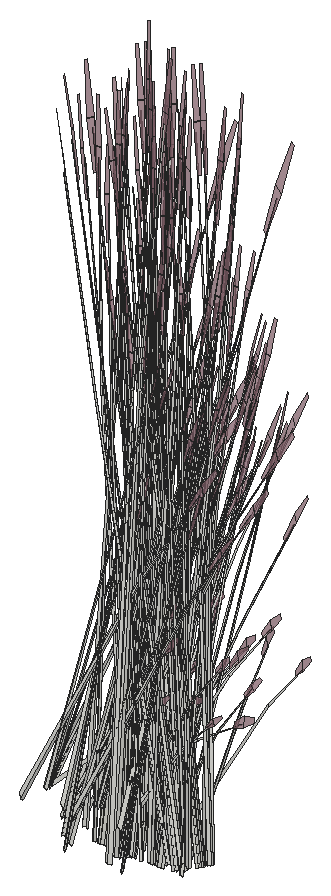
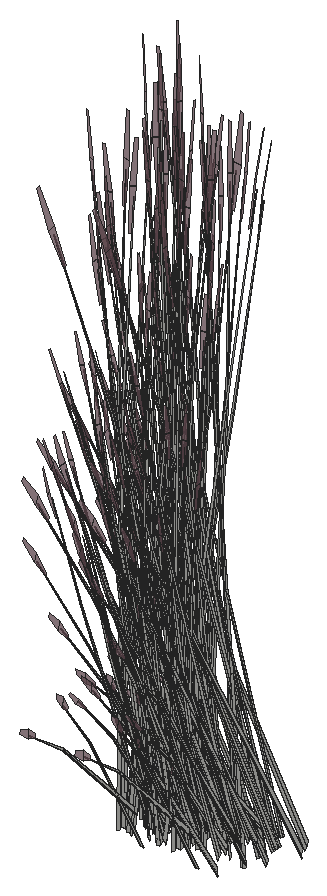
# SketchUp Ruby script. Lengths in inches.
U = 1.inch
M = Sketchup.active_model
def pt(a) = Geom::Point3d.new(a.map { |v| v * U })
def face(e, loops, mat)
  f = e.add_face(loops[0].map { |a| pt(a) })
  loops[1..].each { |l| e.add_face(l.map { |a| pt(a) }).erase! }
  f.material = f.back_material = mat if mat
  f
end
# faces: each face lists its corners as indices into pts; further lists are holes
def faces(e, pts, list, mat = nil) = list.each { |f| face(e, (f[0].is_a?(Array) ? f : [f]).map { |l| l.map { |i| pts[i] } }, mat) }
# xy, xz, yz: faces in a plane at the given z, y or x. An outline is a flat list of corners, or four numbers for a rectangle; further outlines are holes
def ring(l) = l.size == 4 ? [[l[0], l[1]], [l[2], l[1]], [l[2], l[3]], [l[0], l[3]]] : l.each_slice(2).to_a
def flat(e, list, mat, &to3) = list.each { |f| face(e, (f[0].is_a?(Array) ? f : [f]).map { |l| ring(l).map { |u, v| to3.(u, v) } }, mat) }
def xy(e, z, list, mat = nil) = flat(e, list, mat) { |x, y| [x, y, z] }
def xz(e, y, list, mat = nil) = flat(e, list, mat) { |x, z| [x, y, z] }
def yz(e, x, list, mat = nil) = flat(e, list, mat) { |y, z| [x, y, z] }
def lines(e, pts, list) = list.each { |a, b| e.add_line(pt(pts[a]), pt(pts[b])) }
# prism: a flat outline (further loops are holes) pulled along v
def prism(e, loops, v, mat = nil)
  f = face(e, loops, mat); d = Geom::Vector3d.new(v.map { |x| x * U })
  f.pushpull(f.normal.samedirection?(d) ? d.length : -d.length)
end
def box(e, o, s, mat = nil) = prism(e, [[o, [o[0] + s[0], o[1], o[2]], [o[0] + s[0], o[1] + s[1], o[2]], [o[0], o[1] + s[1], o[2]]]], [0, 0, s[2]], mat)
def at(x, y, z, deg = 0) = Geom::Transformation.translation(pt([x, y, z])) * Geom::Transformation.rotation(ORIGIN, Z_AXIS, deg.degrees)
def axes(o, x, y, z) = Geom::Transformation.new([*x, 0, *y, 0, *z, 0, *pt(o).to_a, 1])
def part(name) = M.definitions.add(name)
# library, detail: a bought-in or finely detailed component or shape, given as its bounding box
def library(name, o, s) = part(name).tap { |d| box(d.entities, o, s) }
def detail(e, o, s) = box(e.add_group.entities, o, s)
def put(e, d, t, mat = nil) = e.add_instance(d, t).tap { |i| i.material = mat if mat }
def group(e, t, mat = nil) = e.add_group.tap { |g| g.transformation = t; g.material = mat if mat }.entities
root = M.entities
M.materials.add("LightPink_Translucent").color = [144, 107, 117]
M.materials["LightPink_Translucent"].alpha = 0.75
c1 = part("blade")
p = [[2.15,0.21,22],[0,0.17,0],[0.09,0.45,0],[2.18,0.31,22],[2.29,0.31,22],[0.38,0.45,0],
  [2.48,0.24,33],[2.49,0.24,33],[2.48,0.22,33]]
faces(c1.entities,p,[[0,1,2,3],[4,5,2,3],[6,3,4,7],[8,0,3,6]])
c2 = part("seeds")
p = [[0.3,-0.1,1.38],[-0.01,-0.03,1.59],[-0.01,-0.03,0.03],[0.14,-0.07,-0.07],[0.29,-0.03,3],[0.15,0.01,3.11]]
faces(c2.entities,p,[[0,1,2,3],[1,0,4,5]],"LightPink_Translucent")
c3 = part("blade with seeds")
put(c3.entities,c1,at(0,0,0))
put(c3.entities,c2,axes([2.4,0.25,30.99],[1.5799,-0.05474,1.17369],[-0.12525,1.92788,0.29478],[-0.07173,-0.02425,1.56792]))
put(root,c3,axes([674.73,341.44,393.22],[-0.01592,-0.21915,1.42242],[0.69015,0.14538,0.11501],[-0.04269,0.3123,0.60807]))
put(root,c3,axes([677.3,341.1,393.89],[0.16713,0.52135,-0.42412],[-0.63294,0.0912,-0.32852],[-0.18138,0.14003,0.81151]))
put(root,c3,axes([676.31,342.04,393.91],[-0.01617,0.11299,1.45204],[0.45894,0.39307,-0.22964],[-0.12015,0.18588,0.11645]))
put(root,c3,axes([669.01,340.77,393.22],[-0.24166,-0.09837,1.42242],[0.50011,-0.41269,0.11501],[0.3117,0.18617,0.60807]))
put(root,c3,axes([674.26,340.18,392.06],[0,-0.57097,0.4121],[0.72788,0,0],[0,0.13004,1.30728]))
put(root,c3,axes([674.57,340.71,391.67],[0,0.57097,-0.4121],[-0.72788,0,0],[0,0.13004,1.30728]))
put(root,c3,axes([672.63,342.4375,393.93],[-0.64708,0.13103,0.39842],[-0.1123,-0.514,0.32852],[0.15218,0.15149,0.82444]))
put(root,c3,axes([672.51,342.54,393.93],[-0.29569,0.36271,0.05337],[-0.42107,-0.21117,0.42015],[0.13613,0.11629,0.64067]))
put(root,c3,axes([671.76,341.34,393.22],[-0.14872,-0.18332,1.42242],[0.6872,-0.15433,0.11501],[0.15531,0.28779,0.60807]))
put(root,c3,axes([670.91,340.64,393.93],[0.23895,0.38931,0.05337],[-0.43573,0.19055,0.42015],[0.19208,-0.0376,0.64067]))
put(root,c3,axes([670.33,341.6875,393.76],[0.37017,0.35748,-0.29394],[-0.42268,0.3384,0.37948],[0.21476,0.05149,0.72609]))
put(root,c3,axes([669.91,341.73,394.18],[0.03484,-0.58066,-0.10093],[0.65957,0.01587,-0.56021],[0.25402,0.04034,0.85122]))
put(root,c3,axes([677,340.73,394.18],[0.60181,0.31483,-0.10093],[-0.34671,0.45593,-0.56021],[-0.17003,0.15849,0.85122]))
put(root,c3,axes([670.86,340.51,393.93],[-0.18381,0.5206,0.39842],[-0.60429,-0.17802,0.32852],[0.23764,-0.03129,0.82444]))
put(root,c3,axes([678.36,342.17,391.97],[-0.40676,0.57214,0],[-0.68052,-0.31907,-0.42834],[-0.15499,-0.07267,1.3588]))
put(root,c3,axes([675.77,341.67,391.82],[-0.65588,-0.25634,0],[0.31565,-0.53263,0],[0,0,1.35047]))
put(root,c3,axes([677.29,342.31,391.97],[0.40676,0.57214,0],[-0.68052,0.31907,-0.42834],[-0.15499,0.07267,1.3588]))
put(root,c3,axes([672.53,341.375,391.8125],[0.68303,-0.19373,-0.15934],[0.24001,0.55805,0.00007],[0.07539,-0.02141,1.44335]))
put(root,c3,axes([675.22,342.56,394.2],[-0.64106,-0.14927,0.44225],[0.21921,-0.49074,0.36465],[0.03852,0.19299,0.91512]))
put(root,c3,axes([676.01,342.1,394.6875],[0.5741,0.15241,-0.05385],[-0.1766,0.46909,-0.24415],[-0.0939,0.07122,0.8053]))
put(root,c3,axes([675.05,342.59,393.93],[-0.47939,0.19405,0.05337],[-0.23464,-0.35385,0.42015],[0.0463,0.15598,0.64067]))
put(root,c3,axes([672.41,342.12,394.19],[-0.10048,-0.4599,0.29394],[0.5744,-0.12144,-0.37948],[0.15428,0.13179,0.72609]))
put(root,c3,axes([677.29,340.77,394.19],[0.56631,-0.0816,0.29394],[0.14954,0.46647,-0.37948],[-0.16229,0.12529,0.72609]))
put(root,c3,axes([676.95,341.61,392.05],[0.18794,-0.56744,0.14643],[0.68774,0.16058,0.29122],[-0.1188,0.00276,1.33138]))
put(root,c3,axes([676.63,340.86,392.17],[0.48065,0.34305,0.12018],[-0.40092,0.38703,-0.34318],[-0.1116,0.05232,1.05198]))
put(root,c3,axes([670.48,341.38,393.91],[0.13956,-0.00966,1.45204],[0.38281,-0.44358,-0.22964],[0.24825,0.05855,0.11645]))
put(root,c3,axes([672.54,339.72,391.83],[0.39083,0.47924,-0.37133],[-0.59199,0.33747,0.17871],[0.12647,0.0593,1.19224]))
put(root,c3,axes([677.62,342.99,392.15],[0.2053,-0.09007,1.18691],[0.50689,0.27159,-0.25526],[-0.15087,0.235,0.50747]))
put(root,c3,axes([676.62,340.6,392.26],[0.70648,-0.03525,0.37133],[0.06389,0.58508,-0.17871],[-0.12647,0.0593,1.19224]))
put(root,c3,axes([672.8,339.48,393.71],[-0.56218,-0.29666,1.14775],[0.59361,-0.46189,0.49522],[0.18138,0.27836,1.10941]))
put(root,c3,axes([672.14,340.54,392.3],[-0.40197,0.09426,0.95334],[0.18921,-0.38956,0.70045],[0.21325,0.02666,0.20998]))
put(root,c3,axes([671.85,342.77,393.91],[0.00193,-0.06913,1.47228],[0.55753,-0.30498,-0.13912],[0.19366,0.10886,0.26054]))
put(root,c3,axes([676.79,341.95,391.93],[0.81449,0.18558,0.25528],[-0.20377,0.66335,-0.30288],[-0.13481,0.08302,1.36855]))
put(root,c3,axes([673.65,341.89,392.3],[-0.36631,-0.16417,0.95334],[0.47299,-0.16681,0.70045],[0.12758,0.1413,0.20998]))
put(root,c3,axes([672.35,341.72,392.15],[0.01148,-0.18927,1.18691],[0.54864,-0.21141,-0.25526],[0.16937,0.22654,0.50747]))
put(root,c3,axes([677.14,341.91,392.06],[0.60889,-0.28548,0.4121],[0.36394,0.51192,0],[-0.13868,0.06502,1.30728]))
put(root,c3,axes([679.64,340.8125,392.21],[-0.65687,0.37907,-0.24149],[-0.43681,-0.53562,-0.41502],[-0.16207,-0.0544,1.32557]))
put(root,c3,axes([677.83,342.01,393.93],[-0.46327,-0.38957,0.39842],[0.49199,-0.33598,0.32852],[-0.08546,0.18277,0.82444]))
put(root,c3,axes([675.92,341.45,391.83],[-0.21227,-0.49226,0],[0.60616,-0.17239,0],[0,0,1.28128]))
put(root,c3,axes([675.15,342.48,391.24],[0.10529,-0.03107,1.46364],[0.63335,0.17101,-0.2236],[0.01852,0.19274,0.24931]))
put(root,c3,axes([675.29,342.66,393.76],[-0.19614,0.43908,-0.29394],[-0.57222,-0.12807,0.37948],[0.05247,0.17678,0.72609]))
put(root,c3,axes([669.94,341.45,394.13],[0.65035,0.01375,-0.58968],[-0.04368,0.5789,0.07116],[0.27552,0.06109,0.83415]))
put(root,c3,axes([677.66,341.97,393.93],[-0.53464,-0.0266,0.05337],[0.01466,-0.40172,0.42015],[-0.05594,0.15388,0.64067]))
put(root,c3,axes([673.61,338.65,391.68],[0.15283,0.49751,-0.25712],[-0.60696,0.14127,0.25712],[0.12236,0.05737,1.15348]))
put(root,c3,axes([674.76,340.28,391.97],[0.81352,0,0],[0,0.63814,-0.42834],[0,0.14534,1.3588]))
put(root,c3,axes([677.83,342.13,393.76],[-0.4402,0.30062,-0.29394],[-0.41671,-0.34326,0.37948],[-0.0634,0.1744,0.72609]))
put(root,c3,axes([671.95,342.19,393.91],[-0.05883,-0.04999,1.47228],[0.12868,-0.53581,-0.13912],[0.23172,-0.03423,0.26054]))
put(root,c3,axes([669.52,339.87,393.22],[-0.26985,0.01293,1.42242],[0.17902,-0.56047,0.11501],[0.38456,0.03467,0.60807]))
put(root,c3,axes([673.71,342.64,392.21],[-0.4172,-0.01791,0.872],[0.27552,-0.38032,0.48145],[0.16481,0.13512,0.68401]))
put(root,c3,axes([680.08,341.23,391.71],[-0.43821,0.42916,-0.51753],[-0.54436,-0.38915,-0.13583],[-0.1756,0.10706,1.14236]))
put(root,c3,axes([676.77,340.48,391.83],[-0.31565,0.51449,-0.37133],[-0.65588,-0.24761,0.17871],[0,0.1186,1.19224]))
put(root,c3,axes([676.26,343.2,393.91],[0.07381,-0.03447,1.47228],[0.61004,0.22929,-0.13912],[-0.01434,0.19091,0.26054]))
put(root,c3,axes([674.88,343.4375,393.91],[0.08247,0.09194,1.45204],[0.66552,0.03612,-0.22964],[0.06692,0.20277,0.11645]))
put(root,c3,axes([678.02,340.16,392.05],[-0.51116,-0.4159,0.14643],[0.51512,-0.4034,0.29122],[-0.05645,0.08494,1.33138]))
put(root,c3,axes([680.38,340.99,392.05],[-0.63528,-0.45956,-0.20909],[0.53456,-0.51604,0.45758],[-0.17107,0.05376,1.39619]))
put(root,c3,axes([676.67,340.19,391.9],[0,0.66033,-0.04679],[-0.81352,0,0],[0,0.02075,1.48875]))
put(root,c3,axes([672.36,342.36,394.18],[0.38768,-0.48872,-0.10093],[0.56143,0.28156,-0.56021],[0.19516,0.13808,0.85122]))
put(root,c3,axes([675.22,342.2,394.19],[0.19614,-0.43908,0.29394],[0.57222,0.12807,-0.37948],[0.05247,0.17678,0.72609]))
put(root,c3,axes([678.12,341.81,394.43],[-0.01693,0.52814,-0.65454],[-0.71285,-0.03547,0.07899],[-0.07523,0.22375,0.92591]))
put(root,c3,axes([678.11,343.3,392.3],[-0.01684,-0.3395,0.95334],[0.42072,0.24214,0.70045],[-0.08274,0.16182,0.20998]))
put(root,c3,axes([676.28,341.46,391.9],[0.28286,0.65594,-0.0499],[-0.80821,0.22985,0],[0.00988,0.02291,1.42904]))
put(root,c3,axes([680.06,340.89,391.83],[-0.70648,0.03525,-0.37133],[-0.06389,-0.58508,0.17871],[-0.12647,0.0593,1.19224]))
put(root,c3,axes([672.82,342.12,393.89],[0.64198,-0.13573,-0.42412],[0.1123,0.514,-0.32852],[0.17243,0.1473,0.81151]))
put(root,c3,axes([671.38,341.17,392.15],[-0.15668,-0.14043,1.18691],[0.20386,-0.46454,-0.25526],[0.31701,0.06293,0.50747]))
put(root,c3,axes([675.35,342.26,394.13],[0.31051,0.46426,-0.58968],[-0.63919,0.25873,0.07116],[0.07261,0.22432,0.83415]))
put(root,c3,axes([678.61,340.6,391.83],[-0.81312,-0.00457,-0.0413],[0,-0.63814,0.41452],[-0.02555,0.14527,1.31432]))
put(root,c3,axes([673.56,341.5,394.19],[-0.37017,-0.35748,0.29394],[0.42268,-0.3384,-0.37948],[0.21476,0.05149,0.72609]))
put(root,c3,axes([678.71,341.87,392.06],[0.60889,0.28548,0.4121],[-0.36394,0.51192,0],[-0.13868,-0.06502,1.30728]))
put(root,c3,axes([677.88,342.55,392.79],[0.01429,-0.29475,1.28107],[0.64291,0.15569,0.17703],[-0.0557,0.31414,0.60492]))
put(root,c3,axes([677.02,338.68,392.05],[-0.6991,0.15154,0.14643],[-0.17263,-0.56398,0.29122],[0.06235,0.08217,1.33138]))
put(root,c3,axes([673.89,341.83,393.93],[-0.03276,0.43418,0.05337],[-0.49468,-0.0119,0.42015],[0.18949,0.04543,0.64067]))
put(root,c3,axes([673.75,342.5,391.24],[0.0474,-0.08243,1.46364],[0.59674,-0.24277,-0.2236],[0.18092,0.12565,0.24931]))
put(root,c3,axes([673.94,341.6875,393.93],[-0.47971,0.37622,0.39842],[-0.41372,-0.39954,0.32852],[0.22506,0.0694,0.82444]))
put(root,c3,axes([675.99,343.76,394.6875],[0.44958,-0.32756,-0.05385],[0.41194,0.35875,-0.24415],[0.029,0.10165,0.8053]))
put(root,c3,axes([679.58,340.98,392.17],[-0.12551,0.50956,0.12018],[-0.6132,-0.08845,-0.34318],[-0.1116,-0.05232,1.05198]))
put(root,c3,axes([680.8,342.4,391.67],[-0.60889,0.28548,-0.4121],[-0.36394,-0.51192,0],[-0.13868,0.06502,1.30728]))
put(root,c3,axes([675.1875,341.74,393.26],[-0.12452,-0.47997,-0.02898],[0.58854,-0.11034,-0.1314],[0.1229,0.03043,0.43341]))
put(root,c3,axes([676.79,340.32,391.84],[0.45414,0.3688,0],[-0.45414,0.3688,0],[0,0,1.40491]))
put(root,c3,axes([680.84,342.25,391.82],[-0.40169,-0.57414,-0.04268],[0.68052,-0.31907,0.42834],[-0.16769,0.05466,1.35813]))
put(root,c3,axes([676.79,339.89,392.26],[0.31565,-0.51449,0.37133],[0.65588,0.24761,-0.17871],[0,0.1186,1.19224]))
put(root,c3,axes([676.51,341.68,391.83],[0.65588,0.25634,0],[-0.31565,0.53263,0],[0,0,1.45212]))
put(root,c3,axes([672.89,339.53,391.71],[0.67676,0.09361,-0.51753],[-0.14281,0.57742,-0.13583],[0.20196,0.06997,1.14236]))
put(root,c3,axes([675.58,342.36,393.89],[0.63954,0.14313,-0.42412],[-0.21921,0.49074,-0.32852],[0.05864,0.19758,0.81151]))
put(root,c3,axes([675.03,342.38,394.18],[0.63664,-0.26583,-0.10093],[0.31286,0.47181,-0.56021],[0.084,0.19882,0.85122]))
put(root,c3,axes([678.27,341.99,394.15],[0.46573,0.38364,-0.47077],[-0.49199,0.33598,-0.36465],[-0.07086,0.19492,0.90078]))
put(root,c3,axes([676.57,339.77,391.98],[-0.82229,-0.1203,0.40835],[0.16734,-0.67942,0.16024],[0.12017,0.06561,1.41775]))
put(root,c3,axes([680.66,342.17,391.68],[-0.60696,-0.14127,-0.25712],[0.15283,-0.49751,0.25712],[-0.12236,0.05737,1.15348]))
put(root,c3,axes([678.06,341.7,394.19],[0.4402,-0.30062,0.29394],[0.41671,0.34326,-0.37948],[-0.0634,0.1744,0.72609]))
put(root,c3,axes([678.44,340.7,391.68],[-0.45414,0.35624,-0.25712],[-0.45414,-0.35624,0.25712],[0,0.11474,1.15348]))
put(root,c3,axes([681.01,340.04,392.36],[-0.01777,-0.53759,1.17256],[0.80434,0.13935,0.49647],[-0.19024,0.29416,1.1068]))
put(root,c3,axes([677.15,340.63,391.74],[0.23855,0.52277,-0.57446],[-0.68718,0.18827,-0.15077],[0.02637,0.17702,1.26801]))
put(root,c3,axes([676.81,340.07,391.83],[0.72788,0,0],[0,0.59111,0],[0,0,1.48078]))
put(root,c3,axes([677.78,341.78,394.48],[0.71502,0.02829,-0.11203],[-0.01954,0.53563,-0.62183],[-0.04967,0.20629,0.94486]))
put(root,c3,axes([677.76,342.5625,392.34],[0.59102,-0.10111,0.05401],[0.13587,0.40735,-0.71633],[-0.03747,0.2062,0.64209]))
put(root,c3,axes([677.0625,340.01,392.17],[0.60616,-0.16651,0.12018],[0.21227,0.47548,-0.34318],[0,0.10465,1.05198]))
put(root,c3,axes([680.56,340.73,392.21],[0.07581,0.65151,-0.24149],[-0.7896,0.03939,-0.41502],[-0.13904,0.08678,1.32557]))
put(root,c3,axes([678.8,341.44,393.22],[-0.01592,-0.21915,1.42242],[0.69015,0.14538,0.11501],[-0.04269,0.3123,0.60807]))
put(root,c3,axes([672.75,340.77,393.22],[-0.24166,-0.09837,1.42242],[0.50011,-0.41269,0.11501],[0.3117,0.18617,0.60807]))
put(root,c3,axes([676.85,340.05,392.21],[0.73268,0.27244,-0.24149],[-0.35279,0.57501,-0.41502],[0.02303,0.14118,1.32557]))
put(root,c3,axes([674.66,340.64,393.93],[0.23895,0.38931,0.05337],[-0.43573,0.19055,0.42015],[0.19208,-0.0376,0.64067]))
put(root,c3,axes([674.08,341.6875,393.76],[0.37017,0.35748,-0.29394],[-0.42268,0.3384,0.37948],[0.21476,0.05149,0.72609]))
put(root,c3,axes([673.66,341.73,394.18],[0.03484,-0.58066,-0.10093],[0.65957,0.01587,-0.56021],[0.25402,0.04034,0.85122]))
put(root,c3,axes([674.61,340.51,393.93],[-0.18381,0.5206,0.39842],[-0.60429,-0.17802,0.32852],[0.23764,-0.03129,0.82444]))
put(root,c3,axes([678.44,340.18,392.06],[0,-0.57097,0.4121],[0.72788,0,0],[0,0.13004,1.30728]))
put(root,c3,axes([678.76,340.71,391.67],[0,0.57097,-0.4121],[-0.72788,0,0],[0,0.13004,1.30728]))
put(root,c3,axes([676.8125,342.4375,393.93],[-0.64708,0.13103,0.39842],[-0.1123,-0.514,0.32852],[0.15218,0.15149,0.82444]))
put(root,c3,axes([676.6875,342.54,393.93],[-0.29569,0.36271,0.05337],[-0.42107,-0.21117,0.42015],[0.13613,0.11629,0.64067]))
put(root,c3,axes([675.94,341.34,393.22],[-0.14872,-0.18332,1.42242],[0.6872,-0.15433,0.11501],[0.15531,0.28779,0.60807]))
put(root,c3,axes([679.84,341.67,391.82],[-0.65588,-0.25634,0],[0.31565,-0.53263,0],[0,0,1.35047]))
put(root,c3,axes([681.35,342.31,391.97],[0.40676,0.57214,0],[-0.68052,0.31907,-0.42834],[-0.15499,0.07267,1.3588]))
put(root,c3,axes([674.23,341.38,393.91],[0.13956,-0.00966,1.45204],[0.38281,-0.44358,-0.22964],[0.24825,0.05855,0.11645]))
put(root,c3,axes([679.28,342.56,394.2],[-0.64106,-0.14927,0.44225],[0.21921,-0.49074,0.36465],[0.03852,0.19299,0.91512]))
put(root,c3,axes([676.71,341.375,391.8125],[0.68303,-0.19373,-0.15934],[0.24001,0.55805,0.00007],[0.07539,-0.02141,1.44335]))
put(root,c3,axes([675.88,340.54,392.3],[-0.40197,0.09426,0.95334],[0.18921,-0.38956,0.70045],[0.21325,0.02666,0.20998]))
put(root,c3,axes([679.11,342.59,393.93],[-0.47939,0.19405,0.05337],[-0.23464,-0.35385,0.42015],[0.0463,0.15598,0.64067]))
put(root,c3,axes([681.02,341.61,392.05],[0.18794,-0.56744,0.14643],[0.68774,0.16058,0.29122],[-0.1188,0.00276,1.33138]))
put(root,c3,axes([680.7,340.86,392.17],[0.48065,0.34305,0.12018],[-0.40092,0.38703,-0.34318],[-0.1116,0.05232,1.05198]))
put(root,c3,axes([676.6,342.12,394.19],[-0.10048,-0.4599,0.29394],[0.5744,-0.12144,-0.37948],[0.15428,0.13179,0.72609]))
put(root,c3,axes([680.6875,340.6,392.26],[0.70648,-0.03525,0.37133],[0.06389,0.58508,-0.17871],[-0.12647,0.0593,1.19224]))
put(root,c3,axes([676.73,339.72,391.83],[0.39083,0.47924,-0.37133],[-0.59199,0.33747,0.17871],[0.12647,0.0593,1.19224]))
put(root,c3,axes([680.86,341.95,391.93],[0.81449,0.18558,0.25528],[-0.20377,0.66335,-0.30288],[-0.13481,0.08302,1.36855]))
put(root,c3,axes([676.98,339.48,393.71],[-0.56218,-0.29666,1.14775],[0.59361,-0.46189,0.49522],[0.18138,0.27836,1.10941]))
put(root,c3,axes([673.69,341.45,394.13],[0.65035,0.01375,-0.58968],[-0.04368,0.5789,0.07116],[0.27552,0.06109,0.83415]))
put(root,c3,axes([681.21,341.91,392.06],[0.60889,-0.28548,0.4121],[0.36394,0.51192,0],[-0.13868,0.06502,1.30728]))
put(root,c3,axes([676.04,342.77,393.91],[0.00193,-0.06913,1.47228],[0.55753,-0.30498,-0.13912],[0.19366,0.10886,0.26054]))
put(root,c3,axes([677.83,341.89,392.3],[-0.36631,-0.16417,0.95334],[0.47299,-0.16681,0.70045],[0.12758,0.1413,0.20998]))
put(root,c3,axes([676.53,341.72,392.15],[0.01148,-0.18927,1.18691],[0.54864,-0.21141,-0.25526],[0.16937,0.22654,0.50747]))
put(root,c3,axes([679.99,341.45,391.83],[-0.21227,-0.49226,0],[0.60616,-0.17239,0],[0,0,1.28128]))
put(root,c3,axes([679.22,342.48,391.24],[0.10529,-0.03107,1.46364],[0.63335,0.17101,-0.2236],[0.01852,0.19274,0.24931]))
put(root,c3,axes([675.7,342.19,393.91],[-0.05883,-0.04999,1.47228],[0.12868,-0.53581,-0.13912],[0.23172,-0.03423,0.26054]))
put(root,c3,axes([673.26,339.87,393.22],[-0.26985,0.01293,1.42242],[0.17902,-0.56047,0.11501],[0.38456,0.03467,0.60807]))
put(root,c3,axes([679.36,342.66,393.76],[-0.19614,0.43908,-0.29394],[-0.57222,-0.12807,0.37948],[0.05247,0.17678,0.72609]))
put(root,c3,axes([677.79,338.65,391.68],[0.15283,0.49751,-0.25712],[-0.60696,0.14127,0.25712],[0.12236,0.05737,1.15348]))
put(root,c3,axes([678.9375,340.28,391.97],[0.81352,0,0],[0,0.63814,-0.42834],[0,0.14534,1.3588]))
put(root,c3,axes([680.84,340.48,391.83],[-0.31565,0.51449,-0.37133],[-0.65588,-0.24761,0.17871],[0,0.1186,1.19224]))
put(root,c3,axes([677.89,342.64,392.21],[-0.4172,-0.01791,0.872],[0.27552,-0.38032,0.48145],[0.16481,0.13512,0.68401]))
put(root,c3,axes([678.95,343.4375,393.91],[0.08247,0.09194,1.45204],[0.66552,0.03612,-0.22964],[0.06692,0.20277,0.11645]))
